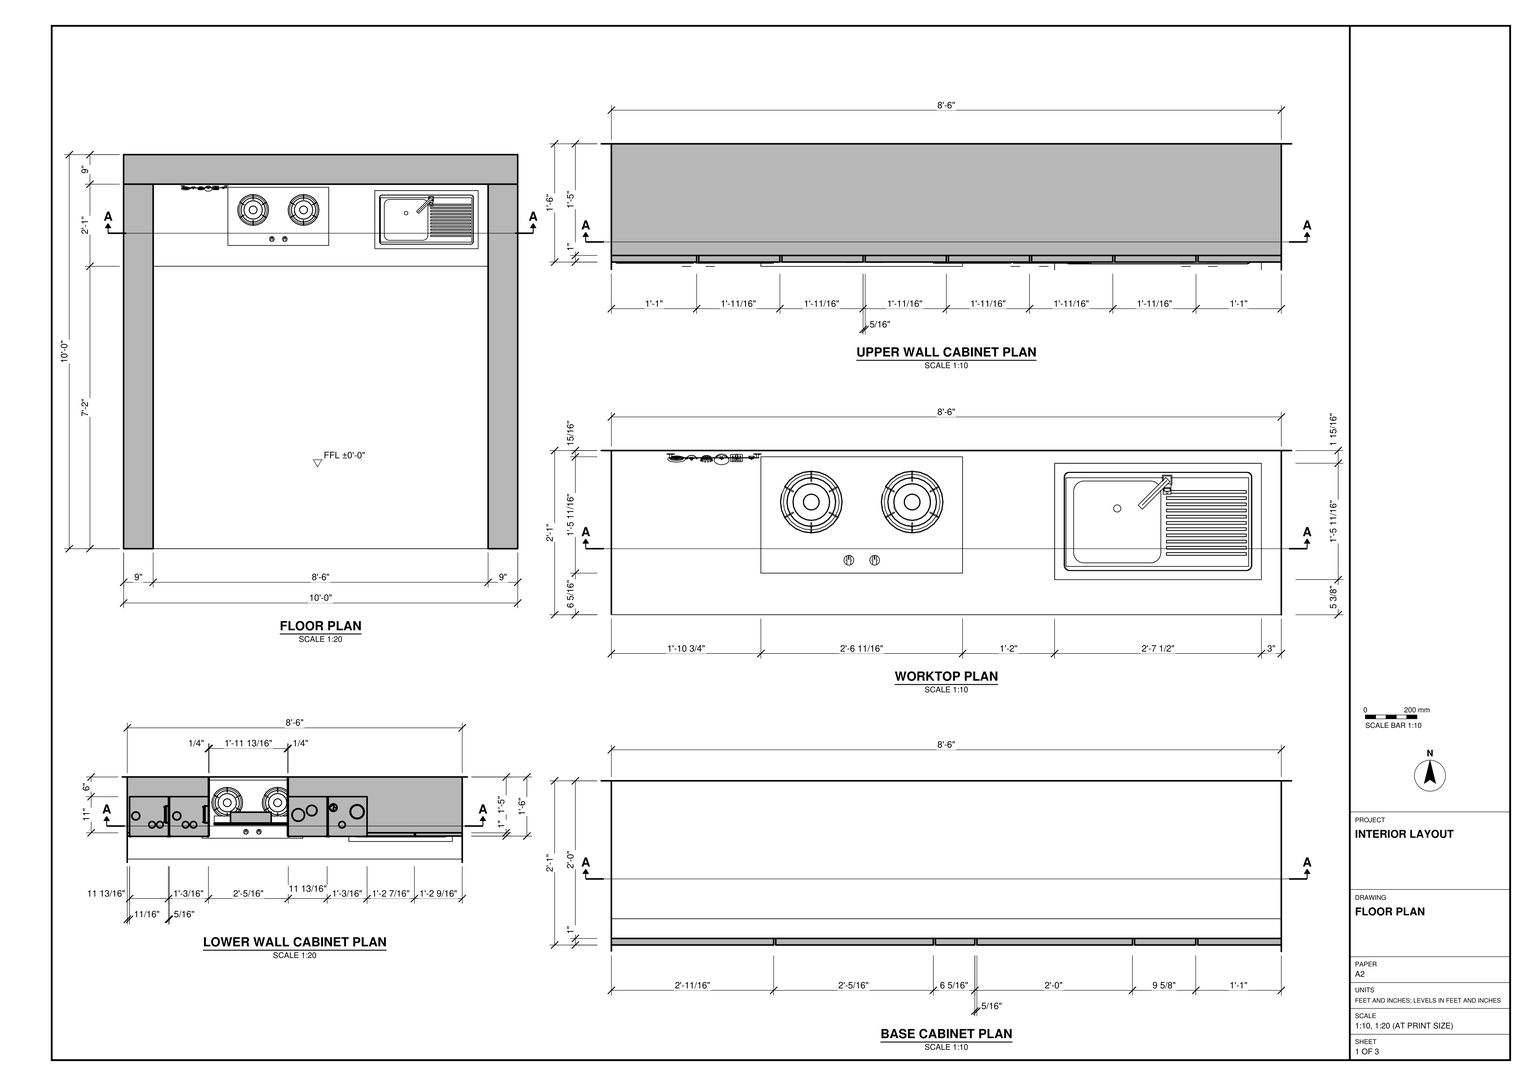
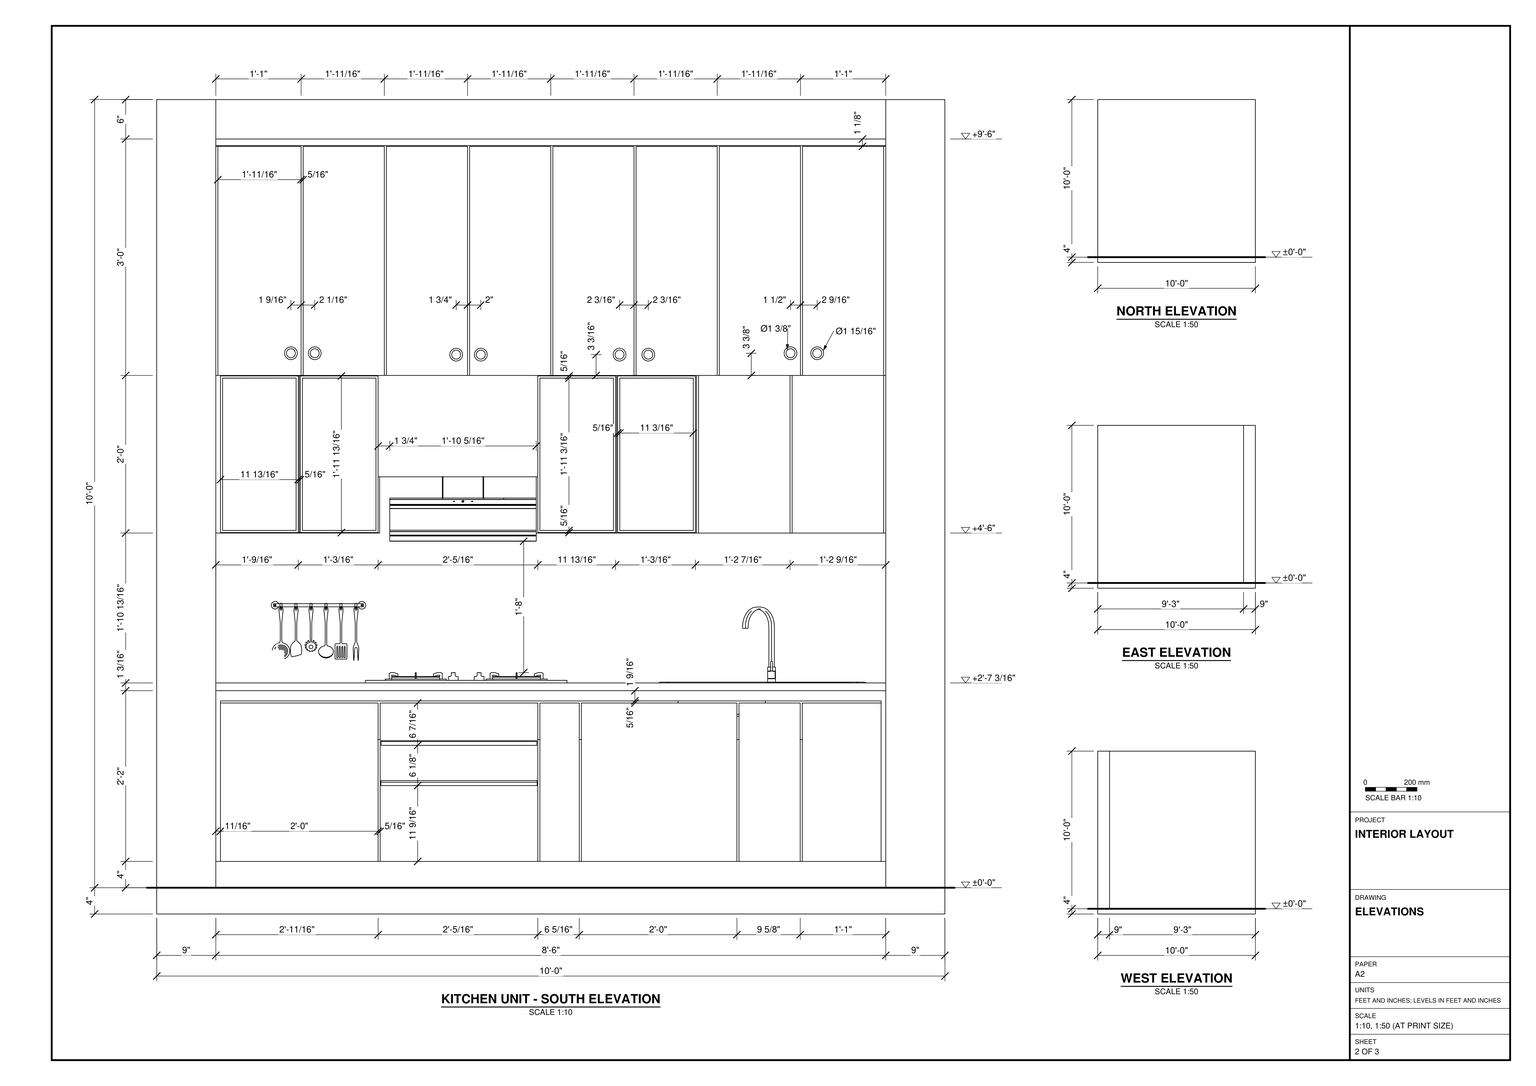
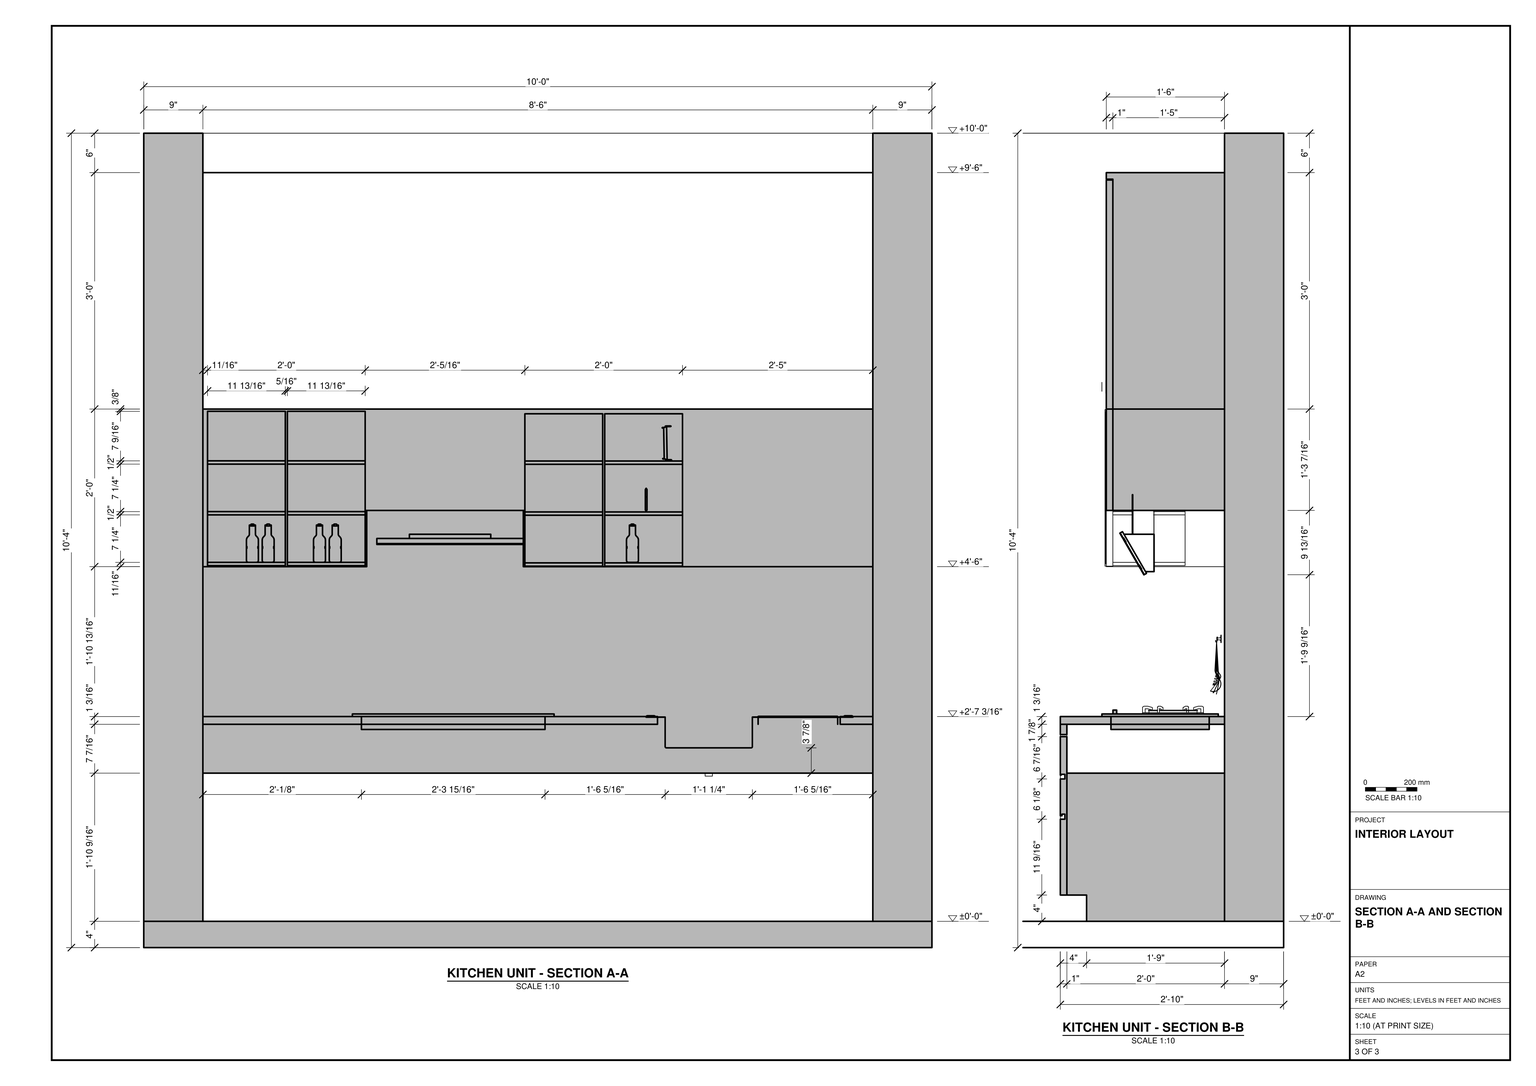
Build the kitchen in SketchUp from task_files/diagram_01.pdf, working in feet and inches. The model is 10'-0" wide, 10'-0" deep and 10'-4" high overall. Set the finished floor at ±0'-0", with the 4" floor slab below it. Form the back wall and two side walls at the drawn 9" thickness, leaving the front open.

Fit the kitchen across the 8'-6" clear width of the back wall. Use the worktop plan to position the cooktop left of centre and the sink with its tap and right-hand drainboard near the right end. Below the worktop, model the cupboard fronts, drawer stack and recessed plinth. Use the south elevation for the cabinet front divisions and the sections for the shelf positions and cabinet depths. Build both tiers of wall cabinets, with the hood aligned over the cooktop and the paired upper doors extending across the run. Place the utensil rail on the wall to the left of the cooktop.

Keep the walls, slab and individual joinery pieces in separate groups or components, and make repeated parts components. Decor, loose items and appliances may be any suitable library components, for example from 3D Warehouse. Save one SketchUp model as output_files/single_wall_kitchen_and_its_room_shell.skp.

# SketchUp Ruby script. Lengths in inches.
U = 1.inch
M = Sketchup.active_model
def pt(a) = Geom::Point3d.new(a.map { |v| v * U })
def face(e, loops, mat)
  f = e.add_face(loops[0].map { |a| pt(a) })
  loops[1..].each { |l| e.add_face(l.map { |a| pt(a) }).erase! }
  f.material = f.back_material = mat if mat
  f
end
# faces: each face lists its corners as indices into pts; further lists are holes
def faces(e, pts, list, mat = nil) = list.each { |f| face(e, (f[0].is_a?(Array) ? f : [f]).map { |l| l.map { |i| pts[i] } }, mat) }
# xy, xz, yz: faces in a plane at the given z, y or x. An outline is a flat list of corners, or four numbers for a rectangle; further outlines are holes
def ring(l) = l.size == 4 ? [[l[0], l[1]], [l[2], l[1]], [l[2], l[3]], [l[0], l[3]]] : l.each_slice(2).to_a
def flat(e, list, mat, &to3) = list.each { |f| face(e, (f[0].is_a?(Array) ? f : [f]).map { |l| ring(l).map { |u, v| to3.(u, v) } }, mat) }
def xy(e, z, list, mat = nil) = flat(e, list, mat) { |x, y| [x, y, z] }
def xz(e, y, list, mat = nil) = flat(e, list, mat) { |x, z| [x, y, z] }
def yz(e, x, list, mat = nil) = flat(e, list, mat) { |y, z| [x, y, z] }
def lines(e, pts, list) = list.each { |a, b| e.add_line(pt(pts[a]), pt(pts[b])) }
# prism: a flat outline (further loops are holes) pulled along v
def prism(e, loops, v, mat = nil)
  f = face(e, loops, mat); d = Geom::Vector3d.new(v.map { |x| x * U })
  f.pushpull(f.normal.samedirection?(d) ? d.length : -d.length)
end
def box(e, o, s, mat = nil) = prism(e, [[o, [o[0] + s[0], o[1], o[2]], [o[0] + s[0], o[1] + s[1], o[2]], [o[0], o[1] + s[1], o[2]]]], [0, 0, s[2]], mat)
def at(x, y, z, deg = 0) = Geom::Transformation.translation(pt([x, y, z])) * Geom::Transformation.rotation(ORIGIN, Z_AXIS, deg.degrees)
def axes(o, x, y, z) = Geom::Transformation.new([*x, 0, *y, 0, *z, 0, *pt(o).to_a, 1])
def part(name) = M.definitions.add(name)
# library, detail: a bought-in or finely detailed component or shape, given as its bounding box
def library(name, o, s) = part(name).tap { |d| box(d.entities, o, s) }
def detail(e, o, s) = box(e.add_group.entities, o, s)
def put(e, d, t, mat = nil) = e.add_instance(d, t).tap { |i| i.material = mat if mat }
def group(e, t, mat = nil) = e.add_group.tap { |g| g.transformation = t; g.material = mat if mat }.entities
root = M.entities
M.materials.add("Brush Stainles Steel").color = [21, 26, 31]
M.materials.add("Material60").color = [0, 0, 8]
M.materials.add("[0136_Charcoal]").color = [35, 35, 35]
M.materials.add("[0137_Black]").color = [0, 0, 0]
M.materials.add("[Carrera Marble]").color = [207, 207, 207]
M.materials.add("[Color_I06]1").color = [12, 0, 204]
M.materials.add("[Translucent Glass Gray]").color = [128, 128, 128]
M.materials["[Translucent Glass Gray]"].alpha = 0.5
M.materials.add("stainless-steel2").color = [0, 0, 0]
c1 = part("Component\#1")
box(c1.entities,[0,0,0],[11.84,11,0.5])
c2 = part("Component\#2")
box(c2.entities,[0,0,0],[11.84,11,0.5])
c3 = library("Knob Handle",[-0.98,-1.57,-0.98],[1.96,1.57,1.96])
c4 = library("Component_12",[0,0,0],[17.72,31.5,20.63])
c5 = part("-   0   +")
prism(c5.entities,[[[0.21,0.4375,-0.06],[0.46,0.4375,-0.06],[0.5,0.39,-0.06],[0.45,0.35,-0.06],[0.2,0.35,-0.06],[0.16,0.39,-0.06]]],[0,0,0.2],"[Color_I06]1")
prism(c5.entities,[[[2.39,0.79,-0.06],[2.65,0.79,-0.06],[2.6875,0.74,-0.06],[2.64,0.69,-0.06],[2.38,0.69,-0.06],[2.34,0.74,-0.06]]],[0,0,0.2],"[Color_I06]1")
prism(c5.entities,[[[2.33,0.09,-0.06],[2.59,0.09,-0.06],[2.625,0.05,-0.06],[2.58,0,-0.06],[2.32,0,-0.06],[2.28,0.05,-0.06]]],[0,0,0.2],"[Color_I06]1")
prism(c5.entities,[[[4.61,0.43,-0.06],[4.67,0.43,-0.06],[4.7,0.39,-0.06],[4.66,0.35,-0.06],[4.6,0.35,-0.06],[4.57,0.39,-0.06]]],[0,0,0.2],"[Color_I06]1")
prism(c5.entities,[[[4.82,0.35,-0.06],[4.75,0.35,-0.06],[4.72,0.39,-0.06],[4.76,0.43,-0.06],[4.82,0.43,-0.06],[4.86,0.39,-0.06]]],[0,0,0.2],"[Color_I06]1")
prism(c5.entities,[[[4.67,0.35,-0.06],[4.71,0.38,-0.06],[4.75,0.35,-0.06],[4.74,0.29,-0.06],[4.7,0.25,-0.06],[4.66,0.29,-0.06]]],[0,0,0.2],"[Color_I06]1")
prism(c5.entities,[[[4.68,0.5,-0.06],[4.72,0.54,-0.06],[4.76,0.5,-0.06],[4.75,0.4375,-0.06],[4.71,0.4,-0.06],[4.68,0.4375,-0.06]]],[0,0,0.2],"[Color_I06]1")
xy(c5.entities,-0.06,[[2.27,0.06,2.23,0.1,2.25,0.35,2.3,0.39,2.35,0.35,2.32,0.1],[2.64,0.06,2.59,0.1,2.62,0.35,2.67,0.39,2.71,0.35,2.6875,0.1],[2.3,0.39,2.26,0.4375,2.28,0.68,2.33,0.73,2.375,0.68,2.36,0.4375],[2.67,0.39,2.625,0.4375,2.65,0.68,2.7,0.73,2.74,0.68,2.72,0.4375]],"[Color_I06]1")
xy(c5.entities,0.14,[[2.27,0.06,2.32,0.1,2.35,0.35,2.3,0.39,2.25,0.35,2.23,0.1],[2.64,0.06,2.6875,0.1,2.71,0.35,2.67,0.39,2.62,0.35,2.59,0.1],[2.3,0.39,2.36,0.4375,2.375,0.68,2.33,0.73,2.28,0.68,2.26,0.4375],[2.67,0.39,2.72,0.4375,2.74,0.68,2.7,0.73,2.65,0.68,2.625,0.4375]],"[Color_I06]1")
p = [[2.23,0.1,-0.06],[2.27,0.06,-0.06],[2.27,0.06,0.14],[2.23,0.1,0.14],[2.25,0.35,-0.06],[2.25,0.35,0.14],
  [2.32,0.1,-0.06],[2.35,0.35,-0.06],[2.35,0.35,0.14],[2.32,0.1,0.14],[2.64,0.06,-0.06],[2.6875,0.1,-0.06],
  [2.6875,0.1,0.14],[2.64,0.06,0.14],[2.59,0.1,-0.06],[2.59,0.1,0.14],[2.62,0.35,-0.06],[2.62,0.35,0.14],
  [2.71,0.35,-0.06],[2.71,0.35,0.14],[2.3,0.39,-0.06],[2.3,0.39,0.14],[2.67,0.39,-0.06],[2.67,0.39,0.14],
  [2.36,0.4375,-0.06],[2.36,0.4375,0.14],[2.26,0.4375,-0.06],[2.26,0.4375,0.14],[2.28,0.68,-0.06],[2.28,0.68,0.14],
  [2.375,0.68,-0.06],[2.375,0.68,0.14],[2.625,0.4375,-0.06],[2.625,0.4375,0.14],[2.65,0.68,-0.06],[2.65,0.68,0.14],
  [2.72,0.4375,-0.06],[2.74,0.68,-0.06],[2.74,0.68,0.14],[2.72,0.4375,0.14],[2.33,0.73,-0.06],[2.33,0.73,0.14],
  [2.7,0.73,-0.06],[2.7,0.73,0.14]]
faces(c5.entities,p,[[0,1,2,3],[4,0,3,5],[6,7,8,9],[1,6,9,2],[10,11,12,13],[14,10,13,15],[16,14,15,17],[11,18,19,12],
  [20,4,5,21],[7,20,21,8],[22,16,17,23],[18,22,23,19],[20,24,25,21],[26,20,21,27],[28,26,27,29],[24,30,31,25],
  [32,22,23,33],[34,32,33,35],[36,37,38,39],[22,36,39,23],[40,28,29,41],[30,40,41,31],[42,34,35,43],[37,42,43,38]],"[Color_I06]1")
c6 = part("komin dół\#1")
prism(c6.entities,[[[9.06,9.76,0],[9.06,9.84,0],[9.92,9.84,0],[9.92,-0.08,0],[-0.08,-0.08,0],[-0.08,9.84,0],[0.79,9.84,0],[0.79,9.76,0],[0.08,9.76,0],[0.08,0.08,0],[9.76,0.08,0],[9.76,9.76,0]]],[0,0,18.125],"stainless-steel2")
c7 = part("komin")
put(c7.entities,c6,at(0,0,0),"Brush Stainles Steel")
c8 = part("korpus")
prism(c8.entities,[[[0,0,17.125],[0,13.78,17.125],[0,13.78,0],[0,9.89,0]]],[19.69,0,0],"stainless-steel2")
c9 = part("panel przód")
yz(c9.entities,0,[[11.02,0,9.65,2.39,9.82,2.49,11.19,0.1],[9.45,2.73,1.57,16.37,1.75,16.47,2.63,14.93,8.34,5.04,8.73,4.36,9.62,2.83],[1.38,16.71,0,19.09,0.17,19.19,1.55,16.81]],"Material60")
yz(c9.entities,0,[[11.19,0.1,9.82,2.49,9.99,2.58,8.9,4.46,8.73,4.36,8.34,5.04,2.63,14.93,2.8,15.03,1.72,16.9,1.55,16.81,0.17,19.19,1.19,19.78,12.22,0.6875]],"stainless-steel2")
yz(c9.entities,35.43,[[11.02,0,11.19,0.1,9.82,2.49,9.65,2.39],[9.45,2.73,9.62,2.83,8.73,4.36,8.34,5.04,2.63,14.93,1.75,16.47,1.57,16.37],[1.38,16.71,1.55,16.81,0.17,19.19,0,19.09]],"Material60")
yz(c9.entities,35.43,[[11.19,0.1,12.22,0.6875,1.19,19.78,0.17,19.19,1.55,16.81,1.72,16.9,2.8,15.03,2.63,14.93,8.34,5.04,8.73,4.36,8.9,4.46,9.99,2.58,9.82,2.49]],"stainless-steel2")
p = [[0,9.65,2.39],[0,11.02,0],[35.43,11.02,0],[35.43,9.65,2.39],[0,11.19,0.1],[35.43,11.19,0.1],
  [0,9.82,2.49],[35.43,9.82,2.49],[0,12.22,0.6875],[35.43,12.22,0.6875],[0,1.19,19.78],[35.43,1.19,19.78],
  [0,9.99,2.58],[35.43,9.99,2.58],[0,8.9,4.46],[35.43,8.9,4.46],[0,1.57,16.37],[0,9.45,2.73],
  [35.43,9.45,2.73],[35.43,1.57,16.37],[0,9.62,2.83],[35.43,9.62,2.83],[0,8.73,4.36],[35.43,8.73,4.36],
  [0,8.34,5.04],[35.43,8.34,5.04],[0,2.63,14.93],[35.43,2.63,14.93],[0,1.75,16.47],[35.43,1.75,16.47],
  [0,2.8,15.03],[35.43,2.8,15.03],[0,1.72,16.9],[35.43,1.72,16.9],[0,0,19.09],[0,1.38,16.71],
  [35.43,1.38,16.71],[35.43,0,19.09],[0,1.55,16.81],[35.43,1.55,16.81],[0,0.17,19.19],[35.43,0.17,19.19]]
faces(c9.entities,p,[[0,1,2,3],[1,4,5,2],[4,6,7,5],[6,0,3,7],[16,17,18,19],[17,20,21,18],[20,22,23,21],[22,24,25,23],
  [24,26,27,25],[26,28,29,27],[28,16,19,29],[34,35,36,37],[35,38,39,36],[38,40,41,39],[40,34,37,41]],"Material60")
faces(c9.entities,p,[[4,8,9,5],[8,10,11,9],[12,6,7,13],[14,12,13,15],[22,14,15,23],[30,26,27,31],[32,30,31,33],[38,32,33,39],
  [10,40,41,11]],"stainless-steel2")
c10 = part("BERG Spring 90")
p = [[27.56,1.88,18.59],[27.56,1.19,19.78]]
lines(c10.entities,p,[[0,1]])
put(c10.entities,c7,at(12.8,5.82,18.59))
put(c10.entities,c8,at(7.875,1.88,1.46))
put(c10.entities,c9,at(0,0,0))
c11 = part("BERG+Spring+90")
put(c11.entities,c5,axes([14.86,0.79,17.53],[0.97787,0,0],[0,-0.48894,0.84686],[0,-0.84686,-0.48894]))
put(c11.entities,c10,axes([0,0,0],[0.97787,0,0],[0,0.97787,0],[0,0,0.97787]))
c12 = library("GAS STOVE",[-0.59,-0.59,-1.97],[30.71,17.72,3.54])
c13 = library("KITCHEN ITEMS (27)",[-13.3,-12.6875,0],[26.6,25.375,20.07])
c14 = library("skpD5F4",[0,-2.85,-0.14],[24.79,2.85,15.53])
c15 = library("78970098",[-130,-130,0],[260,260,30])
c16 = part("Group\#10")
xz(c16.entities,0.1,[[0.32,0.32,11.52,0.32,11.52,23.52,0.32,23.51]],"[Translucent Glass Gray]")
g1 = group(c16.entities,at(0,0,0))
prism(g1,[[[0,0,23.84],[0,0,0],[11.84,0,0],[11.84,0,23.84]],[[0.32,0,23.52],[11.52,0,23.52],[11.52,0,0.32],[0.32,0,0.32]]],[0,0.2,0])
c17 = library("Group\#260",[0,0,0],[30.82,7.02,10])
c18 = library("Group\#245",[0,0,0],[7,7.02,10])
c19 = library("Group\#246",[0,0,0],[7.01,7.02,8.25])
c20 = library("Group\#244",[0,0,0],[7,7.02,8.25])
c21 = library("Group\#243",[0,0,0],[7,7.02,10])
c22 = library("Group\#21",[-1.45,-1.45,0],[9.94,9.94,7.46])
c23 = library("Group77\#2",[-35,-35,0],[70,70,205])
c24 = library("Group\#22",[-1.93,-1.93,0],[13.18,13.18,3.73])
box(root,[33.71,93,58],[0.23,18,8.5625])
box(root,[57.79,93,58],[0.23,18,8.5625])
yz(root,9,[[87,26.5625,111,35.18]])
yz(root,111,[[87,26.5625,111,35.18]])
put(root,c1,at(9.71,94,58.16))
put(root,c1,at(21.87,94,58.16))
put(root,c1,at(21.87,94,65.89))
put(root,c1,at(9.71,94,65.89))
put(root,c1,at(21.87,94,73.61))
put(root,c1,at(9.71,94,73.61))
put(root,c2,at(58.02,94,58.08))
put(root,c2,at(70.18,94,58.08))
put(root,c2,at(70.18,94,65.83))
put(root,c2,at(58.02,94,65.83))
put(root,c2,at(70.18,94,73.59))
put(root,c2,at(58.02,94,73.59))
put(root,c3,at(20.4375,93,85.38))
put(root,c3,at(24.0625,93,85.38))
put(root,c3,at(100.5625,93,85.38))
put(root,c3,at(96.5,93,85.38))
put(root,c3,at(74.84,93,85.17))
put(root,c3,at(70.47,93,85.17))
put(root,c3,at(49.34,93,85.17))
put(root,c3,at(45.59,93,85.17))
put(root,c4,at(76.48,109.0625,26.11,-90))
put(root,c11,axes([35.49,95.0625,56.76],[0.64363,0,0],[0,0.34,0],[0,0,0.34]))
put(root,c12,at(32.35,92.92,35.18))
put(root,c13,axes([18.34,103.12,35.18],[0.3168,0,0],[0,0.3168,0],[0,0,0.3168]))
put(root,c14,axes([17.44,110.51,38.67],[0.58,0,0],[0,0.58,0],[0,0,0.58]))
put(root,c15,axes([31.99,99.59,61.36],[0,-0.02097,0],[-0.00037,0,0.02097],[0.04446,0,0.00078]))
put(root,c15,axes([20.16,99.59,61.36],[0,-0.02097,0],[-0.00037,0,0.02097],[0.04488,0,0.00078]))
put(root,c15,axes([78.97,96.73,76.79],[0,-0.02097,0],[-0.00037,0,0.02097],[0.04446,0,0.00078]))
g2 = group(root,at(0,0,0))
box(g2,[0,0,0],[120,120,4])
g3 = group(root,at(0,111,4))
xy(g3,0,[[0,0,120,9]])
xy(g3,120,[[0,0,120,9]])
xz(g3,0,[[0,0,120,120]],"[Carrera Marble]")
xz(g3,9,[[0,0,120,120]])
yz(g3,0,[[0,0,9,120]])
yz(g3,120,[[0,0,9,120]])
g4 = group(root,at(111,0,4))
box(g4,[0,0,0],[9,111,120])
g5 = group(root,at(0,0,4))
box(g5,[0,0,0],[9,111,120])
g6 = group(root,at(9,87,4))
prism(g6,[[[0,24,0],[0,3,0],[0,3,4],[0,0,4],[0,0,22.5625],[0,24,22.5625]]],[102,0,0])
g7 = group(root,at(9,86,8))
box(g7,[79.65,0,0],[9.33,1,24.12])
box(g7,[49.34,0,0],[6,1,24.12])
box(g7,[55.65,0,0],[23.69,1,24.12])
xy(g7,0,[[0,0,24.71,1],[25.02,0,49.02,1],[89.29,0,102,1]])
xy(g7,11.55,[[25.14,0,48.91,0.7]],"[0136_Charcoal]")
xy(g7,12.07,[[25.14,0,48.91,0.25]],"[0136_Charcoal]")
xy(g7,12.32,[[25.14,0.25,48.91,0.7]],"[0136_Charcoal]")
xy(g7,17.68,[[25.17,0,48.875,0.7]],"[0136_Charcoal]")
xy(g7,18.26,[[25.17,0,48.875,0.125]],"[0136_Charcoal]")
xy(g7,18.38,[[25.17,0.125,48.875,0.7]],"[0136_Charcoal]")
xy(g7,24.12,[[0.71,0,24.71,1],[25.02,0,49.02,1],[89.29,0,101.29,1]])
xy(g7,24.4375,[[0.71,0,101.29,1]])
xy(g7,26,[[0,0,102,1]])
xz(g7,0,[[0,0,0.71,26],[0.71,0,24.71,24.12],[[25.02,0,49.02,24.12],[25.17,17.68,48.875,18.26],[25.14,11.55,48.91,12.07]],[89.29,0,101.29,24.12],[101.29,0,102,26],
  [0.71,24.4375,101.29,26]])
xz(g7,0.125,[[25.17,18.26,48.875,18.38]])
xz(g7,0.25,[[25.14,12.07,48.91,12.32]])
xz(g7,0.7,[[25.14,11.55,48.91,12.32],[25.17,17.68,48.875,18.38]],"[0136_Charcoal]")
xz(g7,1,[[0,0,0,26,102,26,102,0,89.29,0,89.29,24.12,101.29,24.12,101.29,24.4375,0.71,24.4375,0.71,24.12,24.71,24.12,24.71,0],[25.02,0,49.02,24.12]])
yz(g7,0,[[0,0,1,26]])
yz(g7,0.71,[[0,24.12,1,24.4375]])
yz(g7,24.71,[[0,0,1,24.12]])
yz(g7,25.02,[[0,0,1,24.12]])
yz(g7,25.14,[[0,11.55,0.7,11.55,0.7,12.32,0.25,12.32,0.25,12.07,0,12.07]],"[0136_Charcoal]")
yz(g7,25.17,[[0,17.68,0.7,17.68,0.7,18.38,0.125,18.38,0.125,18.26,0,18.26]],"[0136_Charcoal]")
yz(g7,48.875,[[0,17.68,0,18.26,0.125,18.26,0.125,18.38,0.7,18.38,0.7,17.68]],"[0136_Charcoal]")
yz(g7,48.91,[[0,11.55,0,12.07,0.25,12.07,0.25,12.32,0.7,12.32,0.7,11.55]],"[0136_Charcoal]")
yz(g7,49.02,[[0,0,1,24.12]])
yz(g7,89.29,[[0,0,1,24.12]])
yz(g7,101.29,[[0,24.12,1,24.4375]])
yz(g7,102,[[0,0,1,26]])
p = [[24.71,1,0],[25.02,1,0],[49.02,1,0],[49.34,1,0],[55.34,1,0],[55.65,1,0],
  [79.34,1,0],[79.65,1,0],[88.98,1,0],[89.29,1,0]]
lines(g7,p,[[0,1],[2,3],[4,5],[6,7],[8,9]])
g8 = group(root,at(9,94,58))
xy(g8,0,[[0,0,24.71,17],[49.02,0,102,17]])
xy(g8,0.08,[[49.02,0,60.87,11],[61.18,0,73.02,11]])
xy(g8,0.16,[[0.71,0,12.55,11],[12.87,0,24.71,11]])
xy(g8,8.5625,[[24.71,0,49.02,17]])
xy(g8,23.28,[[49.02,0,60.87,11],[61.18,0,73.02,11]])
xy(g8,23.66,[[0.71,0,12.55,11],[12.87,0,24.71,11]])
xy(g8,24,[[0,0,102,17]])
xz(g8,0,[[[0,0,24.71,0,24.71,0.16,12.87,0.16,12.87,23.66,24.71,23.66,24.71,8.5625,49.02,8.5625,49.02,23.28,60.87,23.28,60.87,0.08,49.02,0.08,49.02,0,102,0,102,24,0,24],[0.71,0.16,12.55,23.66],[61.18,0.08,73.02,23.28]]])
xz(g8,11,[[49.02,0.08,60.87,23.28],[61.18,0.08,73.02,23.28],[0.71,0.16,12.55,23.66],[12.87,0.16,24.71,23.66]])
xz(g8,17,[[0,0,0,24,102,24,102,0,49.02,0,49.02,8.5625,24.71,8.5625,24.71,0]])
yz(g8,0,[[0,0,17,24]])
yz(g8,0.71,[[0,0.16,11,23.66]])
yz(g8,12.55,[[0,0.16,11,23.66]])
yz(g8,12.87,[[0,0.16,11,23.66]])
yz(g8,24.71,[[0,0,17,0,17,8.5625,11,8.5625,11,0.16,0,0.16],[0,0.16,11,8.5625],[0,8.5625,11,23.66]])
yz(g8,49.02,[[0,0,0,0.08,11,0.08,11,8.5625,17,8.5625,17,0],[0,0.08,11,8.5625],[0,8.5625,11,23.28]])
yz(g8,60.87,[[0,0.08,11,23.28]])
yz(g8,61.18,[[0,0.08,11,23.28]])
yz(g8,73.02,[[0,0.08,11,23.28]])
yz(g8,102,[[0,0,17,24]])
g9 = group(root,at(9,93,58))
xy(g9,0,[[0,0,24.71,1],[49.02,0,87.43,1],[87.75,0,102,1]])
xy(g9,0.08,[[0.71,0,12.55,1],[12.87,0,24.71,1],[49.02,0,60.87,1],[61.18,0,73.02,1]])
xy(g9,8.5625,[[24.71,0,49.02,1]])
xy(g9,23.92,[[0.71,0,12.55,1],[12.87,0,24.71,1],[49.02,0,60.87,1],[61.18,0,73.02,1]])
xy(g9,24,[[0,0,87.43,1],[87.75,0,102,1]])
xz(g9,0,[[0,0,0.71,24],[0.71,0,12.55,0.08],[12.55,0,12.71,0.08],[12.71,0,12.87,0.08],[12.87,0,24.71,0.08],
  [49.02,0,60.87,0.08],[60.87,0,61.02,24],[61.02,0,61.18,24],[61.18,0,73.02,0.08],[73.02,0,73.18,24],
  [73.18,0,73.5,24],[73.5,0,87.43,24],[87.75,0,101.69,24],[101.69,0,102,24],[12.55,0.08,12.71,23.92],
  [12.71,0.08,12.87,23.92],[24.71,8.5625,49.02,24],[0.71,23.92,24.71,24],[49.02,23.92,60.87,24],[61.18,23.92,73.02,24]])
xz(g9,1,[[[0,0,0,24,87.43,24,87.43,0,49.02,0,49.02,0.08,60.87,0.08,60.87,23.92,49.02,23.92,49.02,8.5625,24.71,8.5625,24.71,23.92,12.87,23.92,12.87,0.08,24.71,0.08,24.71,0],[0.71,0.08,12.55,23.92],[61.18,0.08,73.02,23.92]],[87.43,0,87.75,24],[87.75,0,102,24]])
yz(g9,0,[[0,0,1,24]])
yz(g9,0.71,[[0,0.08,1,23.92]])
yz(g9,12.55,[[0,0.08,1,23.92]])
yz(g9,12.87,[[0,0.08,1,23.92]])
yz(g9,24.71,[[0,0,1,0.08],[0,0.08,1,8.5625],[0,8.5625,1,23.92]])
yz(g9,49.02,[[0,0,1,0.08],[0,0.08,1,8.5625],[0,8.5625,1,23.92]])
yz(g9,60.87,[[0,0.08,1,23.92]])
yz(g9,61.18,[[0,0.08,1,23.92]])
yz(g9,73.02,[[0,0.08,1,23.92]])
yz(g9,87.43,[[0,0,1,24]])
yz(g9,87.75,[[0,0,1,24]])
yz(g9,102,[[0,0,1,24]])
put(root,c16,at(9.71,92.8,58.08))
put(root,c16,at(21.87,92.8,58.08))
put(root,c16,at(58.02,92.8,58.08))
put(root,c16,at(70.18,92.8,58.08))
g10 = group(root,at(9,94,82))
prism(g10,[[[0,17,36],[0,17,0],[0,0,0],[0,0,35],[0,-1,35],[0,-1,36]]],[102,0,0])
g11 = group(root,at(9,93,82))
prism(g11,[[[0,1,0],[12.99,1,0],[12.99,0,0],[0.31,0,0],[0,0,0]]],[0,0,34.875])
prism(g11,[[[89.33,0,0],[89.33,1,0],[102,1,0],[102,0,0],[101.69,0,0]]],[0,0,34.875])
box(g11,[13.3,0,0],[12.36,1,34.875])
box(g11,[25.97,0,0],[12.36,1,34.875])
box(g11,[38.64,0,0],[12.36,1,34.875])
box(g11,[51.31,0,0],[12.36,1,34.875])
box(g11,[63.99,0,0],[12.35,1,34.875])
box(g11,[76.66,0,0],[12.35,1,34.875])
p = [[13.3,1,0],[12.99,1,0],[25.97,1,0],[25.66,1,0],[38.64,1,0],[38.33,1,0],
  [51.31,1,0],[51,1,0],[63.99,1,0],[63.67,1,0],[76.66,1,0],[76.34,1,0],
  [89.33,1,0],[89.01,1,0]]
lines(g11,p,[[0,1],[2,3],[4,5],[6,7],[8,9],[10,11],[12,13]])
g12 = group(root,at(9,87,34))
xy(g12,0,[[[0,-1,102,24],[69.22,6.36,97.03,6.36,97.03,19.86,85.35,19.86,85.35,18.78,83.875,18.78,83.875,19.86,69.22,19.86]]],"[0137_Black]")
xy(g12,1.18,[[84.54,8.0625,96.65,8.45],[84.54,9.01,96.65,9.39],[84.54,9.95,96.65,10.33],[84.54,10.9,96.65,11.28],[84.54,11.84,96.65,12.22],
  [84.54,12.79,96.65,13.17],[84.54,13.73,96.65,14.11],[84.54,14.68,96.65,15.06],[84.54,15.62,96.65,16],[84.54,16.57,96.65,16.95],
  [84.54,17.51,96.65,17.89]])
xy(g12,1.18,[[[0,-1,102,24],[67.49,4.36,98.96,22.05]],[[67.49,4.36,98.96,22.05],[69.22,6.36,69.22,19.86,83.875,19.86,83.875,18.78,85.35,18.78,85.35,19.86,97.03,19.86,97.03,6.36],[83.875,19.86,85.35,20.26]],[[69.74,5.7,96.71,5.7,96.82,5.71,96.93,5.73,97.03,5.76,97.125,5.8125,97.21,5.87,97.29,5.94,97.37,6.02,97.42,6.11,97.47,6.21,97.51,6.3125,97.53,6.42,97.54,6.52,97.54,19.99,97.53,20.08,97.51,20.18,97.48,20.26,97.4375,20.35,97.39,20.43,97.33,20.5,97.26,20.56,97.18,20.61,97.09,20.65,97.01,20.68,96.91,20.7,96.82,20.71,69.63,20.71,69.54,20.7,69.45,20.68,69.36,20.65,69.28,20.61,69.2,20.56,69.13,20.5,69.07,20.43,69.01,20.35,68.97,20.26,68.94,20.18,68.92,20.08,68.92,6.42,68.95,6.3125,68.98,6.21,69.03,6.11,69.09,6.02,69.16,5.94,69.24,5.87,69.33,5.8125,69.43,5.76,69.53,5.73,69.63,5.71],[69.22,6.36,69.22,19.86,83.875,19.86,83.875,20.26,85.35,20.26,85.35,19.86,97.03,19.86,97.03,6.36]],[83.875,18.78,85.35,19.86],[83.875,19.86,85.35,20.26]],"[0137_Black]")
xz(g12,-1,[[0,0,102,1.18]],"[0137_Black]")
xz(g12,6.36,[[69.22,0,97.03,1.18]],"[0137_Black]")
xz(g12,8.0625,[[84.54,0,96.65,1.18]])
xz(g12,8.45,[[84.54,0,96.65,1.18]])
xz(g12,9.01,[[84.54,0,96.65,1.18]])
xz(g12,9.39,[[84.54,0,96.65,1.18]])
xz(g12,9.95,[[84.54,0,96.65,1.18]])
xz(g12,10.33,[[84.54,0,96.65,1.18]])
xz(g12,10.9,[[84.54,0,96.65,1.18]])
xz(g12,11.28,[[84.54,0,96.65,1.18]])
xz(g12,11.84,[[84.54,0,96.65,1.18]])
xz(g12,12.22,[[84.54,0,96.65,1.18]])
xz(g12,12.79,[[84.54,0,96.65,1.18]])
xz(g12,13.17,[[84.54,0,96.65,1.18]])
xz(g12,13.73,[[84.54,0,96.65,1.18]])
xz(g12,14.11,[[84.54,0,96.65,1.18]])
xz(g12,14.68,[[84.54,0,96.65,1.18]])
xz(g12,15.06,[[84.54,0,96.65,1.18]])
xz(g12,15.62,[[84.54,0,96.65,1.18]])
xz(g12,16,[[84.54,0,96.65,1.18]])
xz(g12,16.57,[[84.54,0,96.65,1.18]])
xz(g12,16.95,[[84.54,0,96.65,1.18]])
xz(g12,17.51,[[84.54,0,96.65,1.18]])
xz(g12,17.89,[[84.54,0,96.65,1.18]])
xz(g12,18.78,[[83.875,0,85.35,1.18]],"[0137_Black]")
xz(g12,19.86,[[69.22,0,83.875,1.18],[85.35,0,97.03,1.18]],"[0137_Black]")
xz(g12,24,[[0,0,102,1.18]],"[0137_Black]")
yz(g12,0,[[-1,0,24,1.18]],"[0137_Black]")
yz(g12,69.22,[[6.36,0,19.86,1.18]],"[0137_Black]")
yz(g12,83.875,[[18.78,0,19.86,1.18]],"[0137_Black]")
yz(g12,84.54,[[8.0625,0,8.45,1.18],[9.01,0,9.39,1.18],[9.95,0,10.33,1.18],[10.9,0,11.28,1.18],[11.84,0,12.22,1.18],
  [12.79,0,13.17,1.18],[13.73,0,14.11,1.18],[14.68,0,15.06,1.18],[15.62,0,16,1.18],[16.57,0,16.95,1.18],
  [17.51,0,17.89,1.18]])
yz(g12,85.35,[[18.78,0,19.86,1.18]],"[0137_Black]")
yz(g12,96.65,[[8.0625,0,8.45,1.18],[9.01,0,9.39,1.18],[9.95,0,10.33,1.18],[10.9,0,11.28,1.18],[11.84,0,12.22,1.18],
  [12.79,0,13.17,1.18],[13.73,0,14.11,1.18],[14.68,0,15.06,1.18],[15.62,0,16,1.18],[16.57,0,16.95,1.18],
  [17.51,0,17.89,1.18]])
yz(g12,97.03,[[6.36,0,19.86,1.18]],"[0137_Black]")
yz(g12,102,[[-1,0,24,1.18]],"[0137_Black]")
put(root,c17,at(437.23,104.22,3.89))
put(root,c18,axes([10.37,97.9,58.66],[0.35,0,0],[0,0.35,0],[0,0,0.35]))
put(root,c19,axes([63.57,99.16,58.39],[0.46,0,0],[0,0.46,0],[0,0,0.46]))
put(root,c20,axes([59.15,97.5,58.58],[0.55,0,0],[0,0.55,0],[0,0,0.55]))
put(root,c21,axes([10.68,96.74,66.39],[0.33,0,0],[0,0.33,0],[0,0,0.33]))
put(root,c21,axes([70.6,100.5,58.54],[0.33,0,0],[0,0.33,0],[0,0,0.33]))
put(root,c18,axes([22.87,97.9,58.66],[0.35,0,0],[0,0.35,0],[0,0,0.35]))
put(root,c18,axes([22.87,97.9,74.11],[0.35,0,0],[0,0.35,0],[0,0,0.35]))
put(root,c18,axes([59.67,97.9,66.33],[0.35,0,0],[0,0.35,0],[0,0,0.35]))
put(root,c20,axes([59.15,97.5,74.09],[0.55,0,0],[0,0.55,0],[0,0,0.55]))
put(root,c22,axes([76.76,98.18,58.58],[0.62,0,0],[0,0.62,0],[0,0,0.62]))
put(root,c23,axes([16.54,96.46,58.66],[0.02843,0,0],[0,-0.02843,0],[0,0,0.02843]))
put(root,c23,axes([18.94,96.46,58.66],[0.02843,0,0],[0,-0.02843,0],[0,0,0.02843]))
put(root,c23,axes([26.75,96.46,58.66],[0.02843,0,0],[0,-0.02843,0],[0,0,0.02843]))
put(root,c23,axes([29.15,96.46,58.66],[0.02843,0,0],[0,-0.02843,0],[0,0,0.02843]))
put(root,c23,axes([74.4,96.46,58.66],[0.02843,0,0],[0,-0.02843,0],[0,0,0.02843]))
put(root,c23,axes([64.8125,99.62,66.33],[0.02843,0,0],[0,-0.02843,0],[0,0,0.02843]))
put(root,c24,axes([22.67,98.88,66.39],[0.43,0,0],[0,0.43,0],[0,0,0.43]))
put(root,c24,axes([27.19,96.75,66.39],[0.43,0,0],[0,0.43,0],[0,0,0.43]))
put(root,c24,axes([15.38,96.75,66.39],[0.43,0,0],[0,0.43,0],[0,0,0.43]))
put(root,c24,axes([10.54,97.89,74.11],[0.43,0,0],[0,0.43,0],[0,0,0.43]))
put(root,c24,axes([71.73,97.89,74.11],[0.43,0,0],[0,0.43,0],[0,0,0.43]))
put(root,c21,axes([72.57,101.66,66.33],[0.33,0,0],[0,0.33,0],[0,0,0.33]))
put(root,c23,axes([76.49,97.03,66.33],[0.02843,0,0],[0,-0.02843,0],[0,0,0.02843]))
